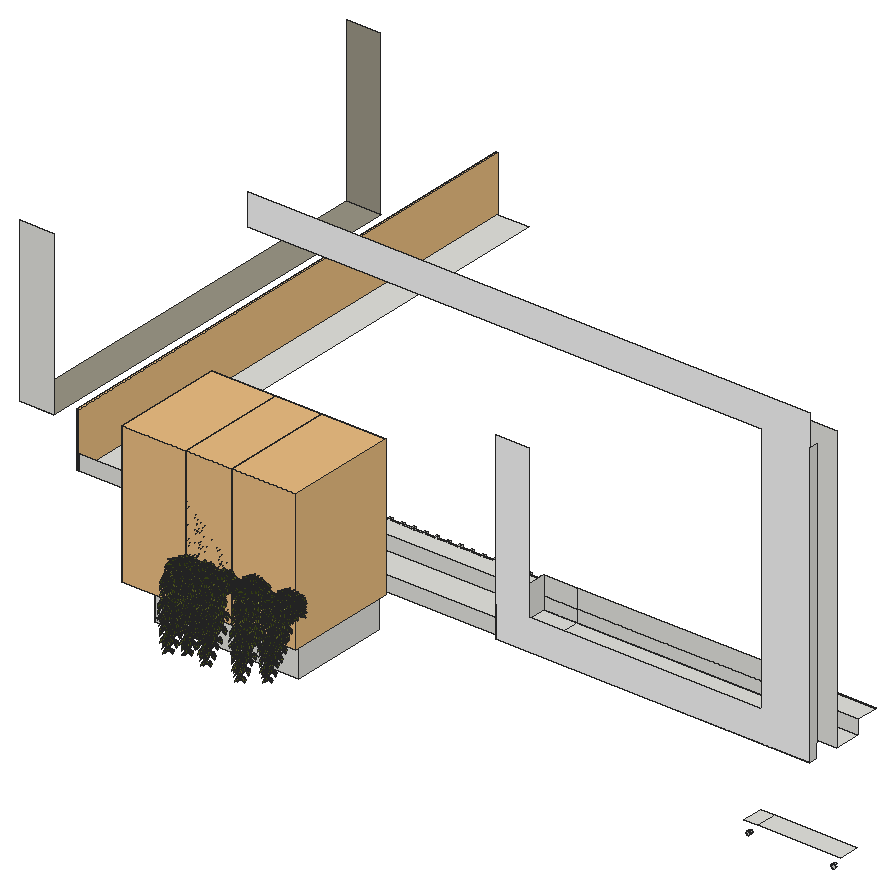
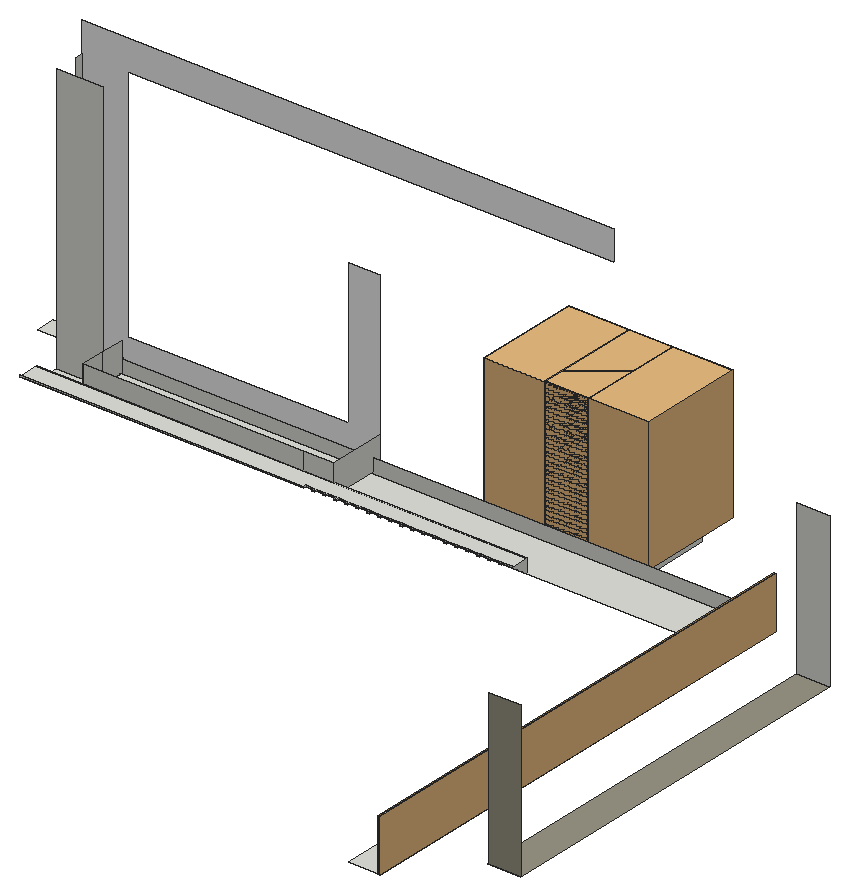
# SketchUp Ruby script. Lengths in inches.
U = 1.inch
M = Sketchup.active_model
def pt(a) = Geom::Point3d.new(a.map { |v| v * U })
def face(e, loops, mat)
  f = e.add_face(loops[0].map { |a| pt(a) })
  loops[1..].each { |l| e.add_face(l.map { |a| pt(a) }).erase! }
  f.material = f.back_material = mat if mat
  f
end
# faces: each face lists its corners as indices into pts; further lists are holes
def faces(e, pts, list, mat = nil) = list.each { |f| face(e, (f[0].is_a?(Array) ? f : [f]).map { |l| l.map { |i| pts[i] } }, mat) }
# xy, xz, yz: faces in a plane at the given z, y or x. An outline is a flat list of corners, or four numbers for a rectangle; further outlines are holes
def ring(l) = l.size == 4 ? [[l[0], l[1]], [l[2], l[1]], [l[2], l[3]], [l[0], l[3]]] : l.each_slice(2).to_a
def flat(e, list, mat, &to3) = list.each { |f| face(e, (f[0].is_a?(Array) ? f : [f]).map { |l| ring(l).map { |u, v| to3.(u, v) } }, mat) }
def xy(e, z, list, mat = nil) = flat(e, list, mat) { |x, y| [x, y, z] }
def xz(e, y, list, mat = nil) = flat(e, list, mat) { |x, z| [x, y, z] }
def yz(e, x, list, mat = nil) = flat(e, list, mat) { |y, z| [x, y, z] }
def lines(e, pts, list) = list.each { |a, b| e.add_line(pt(pts[a]), pt(pts[b])) }
# prism: a flat outline (further loops are holes) pulled along v
def prism(e, loops, v, mat = nil)
  f = face(e, loops, mat); d = Geom::Vector3d.new(v.map { |x| x * U })
  f.pushpull(f.normal.samedirection?(d) ? d.length : -d.length)
end
def box(e, o, s, mat = nil) = prism(e, [[o, [o[0] + s[0], o[1], o[2]], [o[0] + s[0], o[1] + s[1], o[2]], [o[0], o[1] + s[1], o[2]]]], [0, 0, s[2]], mat)
def at(x, y, z, deg = 0) = Geom::Transformation.translation(pt([x, y, z])) * Geom::Transformation.rotation(ORIGIN, Z_AXIS, deg.degrees)
def axes(o, x, y, z) = Geom::Transformation.new([*x, 0, *y, 0, *z, 0, *pt(o).to_a, 1])
def part(name) = M.definitions.add(name)
# library, detail: a bought-in or finely detailed component or shape, given as its bounding box
def library(name, o, s) = part(name).tap { |d| box(d.entities, o, s) }
def detail(e, o, s) = box(e.add_group.entities, o, s)
def put(e, d, t, mat = nil) = e.add_instance(d, t).tap { |i| i.material = mat if mat }
def group(e, t, mat = nil) = e.add_group.tap { |g| g.transformation = t; g.material = mat if mat }.entities
root = M.entities
M.materials.add("[0129_WhiteSmoke]1").color = [245, 245, 245]
M.materials.add("[Concrete Tile]").color = [155, 150, 134]
M.materials.add("asdfasdfasdfasdf").color = [186, 198, 91]
M.materials.add("leaf1_smaller_cleanasdfasfasdfas").color = [88, 95, 33]
M.materials.add("leaf2_smaller_cleansadfasdfasdfasd").color = [55, 66, 19]
c1 = part("glass-railing")
detail(c1.entities,[0,0,0],[1.26,75.59,33.1875])
c2 = library("plant (1)",[-35.72,-28.42,0],[66.31,67.39,84.38])
c3 = part("leaf1a")
p = [[1.06,3.74,11.78],[8.28,8.7,-0.64],[9.51,5.4,26.1],[17.76,4.04,11.26],[17.85,2.23,20],[14.31,3.29,26.73],
  [3.78,3.8125,25.98],[-0.21,2.38,19.72]]
faces(c3.entities,p,[[0,1,2],[2,1,3],[3,4,5],[3,5,2],[6,7,0],[0,2,6]],"leaf1_smaller_cleanasdfasfasdfas")
c4 = part("leaf2a")
p = [[1.4375,3.56,10.81],[8.71,6.8,-0.73],[9.51,3.5,26.59],[16.66,3.91,9.8],[17.86,1.3,19.21],[14.9,1.58,24.92],
  [5.15,2.55,24.01],[1.29,1.87,19.875]]
faces(c4.entities,p,[[0,1,2],[2,1,3],[3,4,5],[3,5,2],[6,7,0],[0,2,6]],"leaf2_smaller_cleansadfasdfasdfasd")
c5 = part("Group\#220")
put(c5.entities,c4,axes([6.68,1.92,2.42],[-0.04671,0.11082,0.08136],[0.07715,0.09226,-0.08136],[-0.11379,0.01705,-0.08856]))
put(c5.entities,c3,axes([1.26,0.54,1.25],[0.13756,-0.04533,0.01029],[0.0079,-0.00888,-0.14471],[0.04581,0.13766,-0.00594]))
put(c5.entities,c4,axes([-0.51,4.89,1.49],[-0.00057,-0.14139,-0.03304],[0.00922,0.03294,-0.14111],[0.14491,-0.00265,0.00885]))
put(c5.entities,c3,axes([4.37,7.98,1.26],[-0.14226,-0.02905,0],[0,0,-0.1452],[0.02905,-0.14226,0]))
put(c5.entities,c3,axes([1.46,4.03,4.07],[0.06242,-0.12847,-0.02614],[-0.10319,-0.03029,-0.09755],[0.08086,0.06051,-0.10432]))
c6 = part("leaf_a")
p = [[1.43,4.41,0.74],[1.39,4.36,0.69],[1.39,4.61,0.21],[1.43,4.67,0.24],[1.35,4.41,0.74],[1.35,4.67,0.24],
  [1.35,3.9,1.02],[1.43,3.9,1.02],[1.39,3.89,0.95],[1.39,3.35,0.9],[1.43,3.34,0.96],[1.35,3.34,0.96]]
faces(c6.entities,p,[[0,1,2,3],[1,4,5,2],[4,0,3,5],[3,2,5],[6,7,0,4],[8,6,4,1],[7,8,1,0],[9,10,11],
  [9,11,6,8],[10,9,8,7],[11,10,7,6]],"asdfasdfasdfasdf")
put(c6.entities,c4,axes([0,-0.08,0.875],[0.1452,0,0],[0,0.02746,-0.14258],[0,0.14258,0.02746]))
c7 = part("leaf_b")
prism(c7.entities,[[[1.36,4.21,-0.25],[1.31,4.13,-0.29],[1.26,4.21,-0.25]]],[0,-0.66,1.14],"asdfasdfasdfasdf")
put(c7.entities,c3,axes([0,-0.1,0.68],[0.1452,-0.0002,0],[0.00006,0.04124,-0.13922],[0.00019,0.13922,0.04124]))
c8 = part("Group\#209")
p = [[2.87,4.13,4.15],[2.98,3.98,4.12],[2.98,4.66,2.59],[2.87,4.8,2.65],[3.09,4.13,4.15],[3.09,4.8,2.65],
  [2.87,4.13,6.07],[2.98,3.98,6.12],[3.09,4.13,6.07],[2.87,5.04,7.34],[2.98,4.91,7.43],[3.09,5.04,7.34]]
faces(c8.entities,p,[[0,1,2,3],[1,4,5,2],[6,7,1,0],[7,8,4,1],[9,10,7,6],[10,11,8,7]],"asdfasdfasdfasdf")
put(c8.entities,c6,axes([0.86,0.51,1.53],[0.95176,-0.27809,0.12967],[0.18405,0.85554,0.48392],[-0.24551,-0.43671,0.86545]))
put(c8.entities,c7,axes([-0.97,2.96,6.52],[0.70711,-0.61237,-0.35355],[0.70711,0.61237,0.35355],[0,-0.5,0.86603]))
put(c8.entities,c6,axes([3.23,0.39,0.41],[0.82736,0.50176,-0.25242],[-0.32519,0.79434,0.5131],[0.45796,-0.34244,0.82037]))
put(c8.entities,c6,axes([3.25,-0.58,4.78],[0.8251,0.44069,-0.35355],[-0.31829,0.8796,0.35355],[0.46679,-0.17918,0.86603]))
c9 = part("Group\#2")
p = [[1.22,4.71,2.14],[1.31,4.57,2.14],[2.16,4.71,3.79],[2.24,4.57,3.77],[1.39,4.71,2.14],[2.33,4.71,3.79],
  [1.93,3.51,6.2],[1.85,3.64,6.23],[2.02,3.64,6.23],[0.93,3.38,8.58],[0.85,3.52,8.58],[1.02,3.52,8.58],
  [0.81,3.57,10.77],[0.72,3.71,10.73],[0.89,3.71,10.73],[1.31,4.57,13.2],[1.22,4.7,13.15],[1.39,4.7,13.15]]
faces(c9.entities,p,[[0,1,2],[3,2,1],[1,4,3],[5,3,4],[6,7,3],[6,3,8],[2,3,7],[5,8,3],
  [9,10,6],[9,6,11],[7,6,10],[8,11,6],[9,11,12],[9,12,10],[13,10,12],[14,12,11],
  [12,15,13],[12,14,15],[16,13,15],[17,15,14]],"asdfasdfasdfasdf")
put(c9.entities,c7,axes([3.93,1.17,1.97],[0.75139,0.49793,0.43299],[-0.65983,0.56085,0.50006],[0.00615,-0.66145,0.74997]))
put(c9.entities,c7,axes([6.23,5.09,1.92],[-0.36585,0.92196,0.12706],[-0.79398,-0.38042,0.47421],[0.48554,0.0726,0.87119]))
put(c9.entities,c7,axes([0.03,0.92,11.26],[1,0,0],[0,0.86603,0.5],[0,-0.5,0.86603]))
put(c9.entities,c6,axes([4.37,2.0625,9.11],[0.45529,0.76896,0.44879],[-0.86129,0.25267,0.44084],[0.22559,-0.58725,0.77733]))
put(c9.entities,c6,axes([1.89,-0.25,4.42],[0.88717,0.14116,0.43931],[-0.36372,0.79981,0.47751],[-0.28396,-0.58342,0.76091]))
put(c9.entities,c6,axes([-0.4,-0.0625,7.9],[0.80178,0.42258,-0.42258],[0,0.70711,0.70711],[0.59763,-0.56694,0.56694]))
put(c9.entities,c7,axes([0.05,0.6875,0.65],[0.97178,0.10445,-0.21151],[0.0126,0.87237,0.48869],[0.23556,-0.47756,0.84643]))
put(c9.entities,c6,axes([5.56,1.19,4.08],[0.24789,0.96746,-0.05068],[-0.86286,0.24427,0.4425],[0.44048,-0.06596,0.89533]))
put(c9.entities,c7,axes([4.91,2.14,7.29],[-0.04249,0.96546,-0.25705],[-0.89911,0.07524,0.4312],[0.43565,0.24944,0.86486]))
c10 = part("Group\#208")
put(c10.entities,c4,axes([5.59,5.52,3.3],[-0.07606,0.12201,-0.02028],[0.09645,0.0436,-0.0994],[-0.07744,-0.06554,-0.10388]))
put(c10.entities,c4,axes([7.69,4.27,1.08],[-0.09839,0.10661,0.00609],[-0.00698,0.00184,-0.14502],[-0.10656,-0.09856,0.00388]))
put(c10.entities,c3,axes([3.51,6.9,2.1],[-0.1403,-0.03711,-0.00465],[-0.00046,0.01976,-0.14385],[0.03739,-0.13898,-0.01921]))
put(c10.entities,c4,axes([2.18,0.07,1.375],[0.14025,0.00096,-0.03757],[-0.03758,0.00358,-0.14021],[0,0.14515,0.00371]))
put(c10.entities,c3,axes([-0.62,2,1.16],[0.081,-0.0806,-0.00996],[0.00004,0.01411,-0.11384],[0.08122,0.08039,0.00999]))
c11 = part("Group\#221")
p = [[1.22,4.71,2.14],[1.31,4.57,2.14],[2.16,4.71,3.79],[2.24,4.57,3.77],[1.39,4.71,2.14],[2.33,4.71,3.79],
  [1.93,3.51,6.2],[1.85,3.64,6.23],[2.02,3.64,6.23],[0.93,3.38,8.58],[0.85,3.52,8.58],[1.02,3.52,8.58],
  [0.81,3.57,10.77],[0.72,3.71,10.73],[0.89,3.71,10.73],[1.31,4.57,13.2],[1.22,4.7,13.15],[1.39,4.7,13.15]]
faces(c11.entities,p,[[0,1,2],[3,2,1],[1,4,3],[5,3,4],[6,7,3],[6,3,8],[2,3,7],[5,8,3],
  [9,10,6],[9,6,11],[7,6,10],[8,11,6],[9,11,12],[9,12,10],[13,10,12],[14,12,11],
  [12,15,13],[12,14,15],[16,13,15],[17,15,14]],"asdfasdfasdfasdf")
put(c11.entities,c7,axes([3.93,1.17,1.97],[0.75139,0.49793,0.43299],[-0.65983,0.56085,0.50006],[0.00615,-0.66145,0.74997]))
put(c11.entities,c7,axes([6.23,5.09,1.92],[-0.36585,0.92196,0.12706],[-0.79398,-0.38042,0.47421],[0.48554,0.0726,0.87119]))
put(c11.entities,c7,axes([0.03,0.92,11.26],[1,0,0],[0,0.86603,0.5],[0,-0.5,0.86603]))
put(c11.entities,c6,axes([4.37,2.0625,9.11],[0.45529,0.76896,0.44879],[-0.86129,0.25267,0.44084],[0.22559,-0.58725,0.77733]))
put(c11.entities,c6,axes([1.89,-0.25,4.42],[0.88717,0.14116,0.43931],[-0.36372,0.79981,0.47751],[-0.28396,-0.58342,0.76091]))
put(c11.entities,c6,axes([-0.4,-0.0625,7.9],[0.80178,0.42258,-0.42258],[0,0.70711,0.70711],[0.59763,-0.56694,0.56694]))
put(c11.entities,c7,axes([0.05,0.6875,0.65],[0.97178,0.10445,-0.21151],[0.0126,0.87237,0.48869],[0.23556,-0.47756,0.84643]))
put(c11.entities,c6,axes([5.56,1.19,4.08],[0.24789,0.96746,-0.05068],[-0.86286,0.24427,0.4425],[0.44048,-0.06596,0.89533]))
put(c11.entities,c7,axes([4.91,2.14,7.29],[-0.04249,0.96546,-0.25705],[-0.89911,0.07524,0.4312],[0.43565,0.24944,0.86486]))
c12 = part("Trailing philodendron")
put(c12.entities,c3,axes([3.65,12.52,19.68],[-0.0527,-0.13492,0.0101],[-0.03487,0.00307,-0.14092],[0.13073,-0.05357,-0.03351]))
put(c12.entities,c3,axes([5.13,11.34,20.6],[-0.03432,-0.12484,0.06572],[-0.08608,-0.03507,-0.11155],[0.11179,-0.06533,-0.06572]))
put(c12.entities,c4,axes([2.61,13.04,18.63],[0.05838,-0.12752,0.03758],[0.01564,-0.03417,-0.14025],[0.13202,0.06044,0]))
put(c12.entities,c4,axes([3.7,9.83,20.73],[-0.00129,-0.14519,0],[-0.0726,0.00064,-0.12575],[0.12574,-0.00112,-0.0726]))
put(c12.entities,c4,axes([11.375,11.11,20.23],[-0.14171,0.00126,0.03163],[-0.02867,0.05638,-0.1307],[-0.01341,-0.1338,-0.05478]))
put(c12.entities,c3,axes([2.4375,12.45,15.12],[-0.02375,-0.14324,0],[0.13106,-0.02173,-0.05859],[0.05781,-0.00958,0.13285]))
put(c12.entities,c3,axes([9.62,10.68,22.01],[0.05693,0.12487,-0.04742],[0.05061,-0.06787,-0.11796],[-0.12361,0.02972,-0.07014]))
put(c12.entities,c3,axes([11.63,16.35,20.5625],[-0.12691,-0.00762,0.07014],[-0.06947,0.03872,-0.12148],[-0.01233,-0.13973,-0.03749]))
put(c12.entities,c3,axes([12.51,17.52,17.81],[-0.1445,0.01001,0.0102],[-0.01383,-0.07182,-0.12544],[-0.0036,-0.1258,0.07242]))
put(c12.entities,c4,axes([9.09,6.34,22.72],[-0.09269,-0.05068,-0.09962],[-0.03661,0.13604,-0.03515],[0.1056,0.00268,-0.09962]))
put(c12.entities,c3,axes([4.83,12.62,22.54],[0.10783,0.09684,-0.00888],[0.09716,-0.10783,0.00397],[-0.00394,-0.00889,-0.14487]))
put(c12.entities,c3,axes([4.94,9.48,20.375],[0.01323,0.07633,0.07653],[0.10803,-0.00667,-0.01203],[-0.00375,0.07738,-0.07653]))
put(c12.entities,c4,axes([14,13.64,21.84],[-0.01852,-0.13907,0.03741],[-0.14373,0.01547,-0.01367],[0.00911,-0.03878,-0.13963]))
put(c12.entities,c4,axes([9.23,4.15,18.71],[0.14198,0.00177,-0.03038],[-0.02867,0.05638,-0.1307],[0.01021,0.13379,0.05548]))
put(c12.entities,c4,axes([5.82,4.5625,15.3],[0.13095,-0.05433,0.03137],[0.06268,0.11013,-0.07089],[0.00273,0.07747,0.12278]))
put(c12.entities,c5,axes([6.59,5.29,16.06],[1.23201,0.26412,0],[-0.26412,1.23201,0],[0,0,1.26]))
put(c12.entities,c8,axes([12.21,1.69,0.66],[-0.82914,0.03045,-0.02227],[0.02366,0.80139,0.21474],[-0.02938,-0.21389,0.80143]))
put(c12.entities,c9,axes([6.8125,1.15,7.57],[0.74375,-0.41052,0.02847],[0.41052,0.73612,-0.11],[0.02847,0.11,0.84237]))
put(c12.entities,c8,axes([-1.68,6.875,13.2],[0.5,-0.86603,0],[0.81585,0.47103,-0.33545],[0.29051,0.16773,0.94206]))
put(c12.entities,c8,axes([1.86,19.56,12.8125],[0.88164,0.4704,0.03781],[0.46333,-0.8476,-0.25863],[0.08962,-0.24554,0.96524]))
g1 = group(c12.entities,at(9.13,11.13,20.67))
put(g1,c4,axes([7.36,4.03,-0.3],[-0.05057,0.11966,-0.06487],[0.07036,-0.03625,-0.12173],[-0.11651,-0.07383,-0.04536]))
put(g1,c4,axes([8.4,1.56,-2.35],[-0.06703,0.12496,-0.03122],[-0.04831,-0.05702,-0.12449],[-0.1194,-0.04708,0.0679]))
put(g1,c3,axes([5.37,5.58,-2.1],[-0.14013,0.0124,0.03596],[-0.03803,-0.04347,-0.13322],[-0.00061,-0.13798,0.0452]))
put(g1,c4,axes([2.45,-0.07,0.8],[0.12002,-0.06072,-0.05468],[-0.07506,-0.04353,-0.11642],[0.03229,0.1245,-0.06737]))
put(g1,c3,axes([0.19,2.38,0.125],[0.05529,-0.09889,0.01797],[-0.03005,-0.03583,-0.10474],[0.09591,0.04578,-0.04318]))
put(c12.entities,c10,axes([17.33,10.54,16.15],[-0.62797,0.46654,0.62289],[-0.59637,-0.80271,0],[0.5,-0.37147,0.78231]))
put(c12.entities,c5,axes([3.44,11.88,17.73],[0.78616,-0.36326,0.5],[0.52263,0.82256,-0.22414],[-0.32986,0.43753,0.83652]))
put(c12.entities,c10,axes([5.5,5.07,16.54],[0.96593,-0.11102,0.2338],[0,0.90334,0.42894],[-0.25882,-0.41432,0.87255]))
put(c12.entities,c8,axes([18.84,3.62,12.91],[-0.80696,-0.59061,0],[-0.57048,0.77946,-0.25882],[-0.15286,0.20886,0.96593]))
put(c12.entities,c9,axes([3.89,0.96,5.21],[0.83948,0.00528,-0.02906],[-0.009,0.83292,-0.10846],[0.02813,0.1087,0.83246]))
put(c12.entities,c9,axes([6.1,0.84,-5.33],[0.875,-0.48296,0.03349],[0.48296,0.86603,-0.12941],[0.03349,0.12941,0.99103]))
put(c12.entities,c9,axes([3.87,-0.55,-8.84],[0.99938,0.00629,-0.0346],[-0.01071,0.99157,-0.12912],[0.03349,0.12941,0.99103]))
put(c12.entities,c8,axes([0.46,6.875,13.01],[0.5,-0.86603,0],[0.81585,0.47103,-0.33545],[0.29051,0.16773,0.94206]))
put(c12.entities,c9,axes([10.39,0.84,1.73],[0.875,-0.48296,0.03349],[0.48296,0.86603,-0.12941],[0.03349,0.12941,0.99103]))
put(c12.entities,c9,axes([-0.75,1.13,2.67],[0.7525,-0.41535,0.0288],[0.41535,0.74478,-0.11129],[0.0288,0.11129,0.85228]))
put(c12.entities,c9,axes([0.04,-0.97,-8.67],[0.735,-0.40569,0.02813],[0.40569,0.72746,-0.1087],[0.02813,0.1087,0.83246]))
put(c12.entities,c9,axes([0.09,-0.6,-7.42],[0.47403,-0.32078,-0.33698],[0.20171,0.57521,-0.26383],[0.41925,0.08595,0.50794]))
put(c12.entities,c9,axes([10.35,0.97,-6.0625],[0.76125,-0.42018,0.02914],[0.42018,0.75344,-0.11259],[0.02914,0.11259,0.86219]))
put(c12.entities,c9,axes([10.78,-1.55,-11.77],[0.72777,-0.42018,0.22517],[0.435,0.75344,0],[-0.19501,0.11259,0.84036]))
put(c12.entities,c9,axes([5.78,-1.55,-20.23],[0.76125,-0.42018,0.02914],[0.42018,0.75344,-0.11259],[0.02914,0.11259,0.86219]))
put(c12.entities,c9,axes([8.72,-1.43,-13.97],[0.65467,-0.36135,0.02506],[0.36135,0.64796,-0.09682],[0.02506,0.09682,0.74149]))
put(c12.entities,c11,axes([1.53,-0.97,-19.86],[0.735,-0.40569,0.02813],[0.40569,0.72746,-0.1087],[0.02813,0.1087,0.83246]))
put(c12.entities,c11,axes([6.23,-2.02,-7.18],[0.55125,-0.30427,0.0211],[0.39555,0.70927,-0.10599],[0.0211,0.08153,0.62435]))
put(c12.entities,c11,axes([6.43,-1.89,6.18],[0.735,-0.40569,0.02813],[0.5274,0.9457,-0.14132],[0.02813,0.1087,0.83246]))
put(c12.entities,c11,axes([10.24,1.09,9.64],[0.62475,-0.34484,0.02391],[0.44829,0.80384,-0.12012],[0.02391,0.0924,0.70759]))
put(c12.entities,c8,axes([1.56,7.74,12.8125],[-0.22619,0.97335,0.03781],[0.93864,0.22817,-0.25863],[0.26037,0.02301,0.96524]))
put(c12.entities,c8,axes([0.65,14.36,12.8125],[0.30411,0.95189,0.03781],[0.92309,-0.28464,-0.25863],[0.23543,-0.11355,0.96524]))
put(c12.entities,c8,axes([7.75,10.38,12.8125],[-0.84074,0.54011,0.03781],[0.51385,0.81797,-0.25863],[0.17062,0.19802,0.96524]))
put(c12.entities,c8,axes([12.92,19.16,12.8125],[0.9234,-0.38197,0.03781],[-0.36017,-0.89632,-0.25863],[-0.13268,-0.22521,0.96524]))
put(c12.entities,c8,axes([6.55,17.22,12.8125],[0.7985,0.60081,0.03781],[0.58857,-0.76596,-0.25863],[0.12643,-0.22877,0.96524]))
put(c12.entities,c8,axes([16.24,8.94,12.8125],[-0.64953,-0.75939,0.03781],[-0.7404,0.62041,-0.25863],[-0.17295,0.19599,0.96524]))
put(c12.entities,c8,axes([15.6875,15.74,12.8125],[0.12972,-0.99083,0.03781],[-0.95648,-0.13509,-0.25863],[-0.26137,0.00261,0.96524]))
put(c12.entities,c8,axes([19.85,8,15.61],[-0.64953,-0.75939,0.03781],[-0.7404,0.62041,-0.25863],[-0.17295,0.19599,0.96524]))
put(c12.entities,c8,axes([18.86,17.5,12.8125],[0.62831,-0.77705,0.03781],[-0.74495,-0.61494,-0.25863],[-0.22422,-0.13434,0.96524]))
put(c12.entities,c8,axes([-0.43,13.28,13.2],[-0.41945,-0.90778,0],[0.85518,-0.39515,-0.33545],[0.30452,-0.14071,0.94206]))
put(c12.entities,c11,axes([4.5625,-2.01,7.45],[0.56595,-0.31238,0.02166],[0.40609,0.72819,-0.10881],[0.02166,0.0837,0.641]))
put(c12.entities,c11,axes([4.48,-2.02,-24.24],[0.55125,-0.30427,0.0211],[0.39555,0.70927,-0.10599],[0.0211,0.08153,0.62435]))
put(c12.entities,c11,axes([4.9,-4.23,-11.04],[0.55125,-0.30427,0.0211],[0.39555,0.70927,-0.10599],[0.0211,0.08153,0.62435]))
put(c12.entities,c10,axes([17.33,10.54,17.41],[-0.62797,0.46654,0.62289],[-0.59637,-0.80271,0],[0.5,-0.37147,0.78231]))
put(c12.entities,c8,axes([-0.03,6.82,20.63],[0.44714,-0.87214,-0.19857],[0.53417,0.43844,-0.7228],[0.71744,0.21712,0.66191]))
put(c12.entities,c8,axes([20.82,12.8,12.8125],[0.12972,-0.99083,0.03781],[-0.95648,-0.13509,-0.25863],[-0.26137,0.00261,0.96524]))
xy(root,138.0625,[[848.72,801.78,857.125,814.22],[857.125,801.78,906.77,814.22]])
xy(root,138.1875,[[514,776.37,600.89,836.7]])
xy(root,153.5625,[[411.09,846.1,827.91,846.1,827.91,861.24,857.125,861.24,857.125,877.14,431.5,877.14,431.5,1160.85,411.09,1160.85]])
xy(root,154.75,[[667.84,840.97,687.49,877.14],[687.49,840.97,827.91,877.14],[827.91,840.97,857.125,845.35]])
xy(root,156.5,[[352.17,877.14,372.92,1122.97]],"[Concrete Tile]")
xy(root,162.125,[[545.16,877.14,545.16,888.95,550.57,888.95,550.57,890.39,552.22,890.39,552.22,888.95,557.63,888.95,557.63,890.39,559.22,890.39,559.22,888.95,564.63,888.95,564.63,890.39,566.22,890.39,566.22,888.95,571.63,888.95,571.63,890.39,573.22,890.39,573.22,888.95,578.63,888.95,578.63,890.39,580.22,890.39,580.22,888.95,585.63,888.95,585.63,890.39,587.22,890.39,587.22,888.95,592.63,888.95,592.63,890.39,594.22,890.39,594.22,888.95,599.63,888.95,599.63,890.39,601.22,890.39,601.22,888.95,606.63,888.95,606.63,890.39,608.22,890.39,608.22,888.95,613.63,888.95,613.63,890.39,615.22,890.39,615.22,888.95,620.63,888.95,620.63,890.39,622.22,890.39,622.22,888.95,627.63,888.95,627.63,890.39,629.22,890.39,629.22,888.95,634.63,888.95,634.63,890.39,636.22,890.39,636.22,888.83,641.63,888.83,641.63,890.39,643.22,890.39,643.22,888.83,648.63,888.83,648.63,890.39,650.22,890.39,650.22,888.83,655.63,888.83,655.63,890.39,657.22,890.39,657.22,888.83,662.63,888.83,662.63,890.39,664.22,890.39,664.22,888.83,669.63,888.83,669.63,890.39,671.22,890.39,671.22,888.83,676.63,888.83,676.63,890.39,857.125,890.39,857.125,877.14]])
xz(root,776.37,[[514,138.1875,600.89,183.3125]])
xz(root,799.91,[[852.61,131.88,852.9,131.92,853.17,132.03,853.4,132.21,853.58,132.44,853.69,132.71,853.73,133,853.69,133.29,853.58,133.57,853.4,133.8,853.17,133.98,852.9,134.09,852.61,134.13,852.32,134.09,852.05,133.98,851.8125,133.8,851.63,133.57,851.52,133.29,851.48,133,851.52,132.71,851.63,132.44,851.8125,132.21,852.05,132.03,852.32,131.92],[903.73,131.88,904.02,131.92,904.3,132.03,904.53,132.21,904.71,132.44,904.82,132.71,904.86,133,904.82,133.29,904.71,133.57,904.53,133.8,904.3,133.98,904.02,134.09,903.73,134.13,903.44,134.09,903.17,133.98,902.9375,133.8,902.76,133.57,902.65,133.29,902.61,133,902.65,132.71,902.76,132.44,902.9375,132.21,903.17,132.03,903.44,131.92]])
xz(root,836.7,[[514,138.1875,600.89,183.3125]])
xz(root,840.97,[[667.84,154.75,857.125,154.75,857.125,343.4375,518.47,343.4375,518.47,324.5625,827.91,324.5625,827.91,173.4375,687.49,173.4375,687.49,264.75,667.84,264.75]],"[0129_WhiteSmoke]1")
xz(root,845.35,[[827.91,154.75,857.125,163]])
xz(root,846.1,[[411.09,153.5625,827.91,162.75]])
xz(root,861.24,[[827.91,153.5625,857.125,324.5625]])
xz(root,877.14,[[545.16,153.5625,857.125,153.5625,857.125,162.125,827.91,162.125,827.91,154.75,667.84,154.75,667.84,162.125,545.16,162.125],[667.84,154.75,687.49,162.125],[687.49,154.75,827.91,162.125],[352.17,156.5,372.92,254.125],[667.84,162.125,687.49,173.4375],
  [687.49,162.125,827.91,173.4375]])
xz(root,888.83,[[636.22,162.125,641.63,162.75],[643.22,162.125,648.63,162.75],[650.22,162.125,655.63,162.75],[657.22,162.125,662.63,162.75],[664.22,162.125,669.63,162.75],
  [671.22,162.125,676.63,162.75]])
xz(root,888.95,[[545.16,162.125,550.57,162.75],[552.22,162.125,557.63,162.75],[559.22,162.125,564.63,162.75],[566.22,162.125,571.63,162.75],[573.22,162.125,578.63,162.75],
  [580.22,162.125,585.63,162.75],[587.22,162.125,592.63,162.75],[594.22,162.125,599.63,162.75],[601.22,162.125,606.63,162.75],[608.22,162.125,613.63,162.75],
  [615.22,162.125,620.63,162.75],[622.22,162.125,627.63,162.75],[629.22,162.125,634.63,162.75]])
xz(root,890.39,[[550.57,162.125,552.22,162.75],[557.63,162.125,559.22,162.75],[564.63,162.125,566.22,162.75],[571.63,162.125,573.22,162.75],[578.63,162.125,580.22,162.75],
  [585.63,162.125,587.22,162.75],[592.63,162.125,594.22,162.75],[599.63,162.125,601.22,162.75],[606.63,162.125,608.22,162.75],[613.63,162.125,615.22,162.75],
  [620.63,162.125,622.22,162.75],[627.63,162.125,629.22,162.75],[634.63,162.125,636.22,162.75],[641.63,162.125,643.22,162.75],[648.63,162.125,650.22,162.75],
  [655.63,162.125,657.22,162.75],[662.63,162.125,664.22,162.75],[669.63,162.125,671.22,162.75],[676.63,162.125,679.76,162.75],[679.76,162.125,857.125,162.75]])
xz(root,1122.97,[[352.17,156.5,372.3,254.125]],"[Concrete Tile]")
yz(root,514,[[776.37,138.1875,836.7,183.3125]])
yz(root,550.57,[[888.95,162.125,890.39,162.75]])
yz(root,552.22,[[888.95,162.125,890.39,162.75]])
yz(root,557.63,[[888.95,162.125,890.39,162.75]])
yz(root,559.22,[[888.95,162.125,890.39,162.75]])
yz(root,564.63,[[888.95,162.125,890.39,162.75]])
yz(root,566.22,[[888.95,162.125,890.39,162.75]])
yz(root,571.63,[[888.95,162.125,890.39,162.75]])
yz(root,573.22,[[888.95,162.125,890.39,162.75]])
yz(root,578.63,[[888.95,162.125,890.39,162.75]])
yz(root,580.22,[[888.95,162.125,890.39,162.75]])
yz(root,585.63,[[888.95,162.125,890.39,162.75]])
yz(root,587.22,[[888.95,162.125,890.39,162.75]])
yz(root,592.63,[[888.95,162.125,890.39,162.75]])
yz(root,594.22,[[888.95,162.125,890.39,162.75]])
yz(root,599.63,[[888.95,162.125,890.39,162.75]])
yz(root,600.89,[[776.37,138.1875,836.7,183.3125]])
yz(root,601.22,[[888.95,162.125,890.39,162.75]])
yz(root,606.63,[[888.95,162.125,890.39,162.75]])
yz(root,608.22,[[888.95,162.125,890.39,162.75]])
yz(root,613.63,[[888.95,162.125,890.39,162.75]])
yz(root,615.22,[[888.95,162.125,890.39,162.75]])
yz(root,620.63,[[888.95,162.125,890.39,162.75]])
yz(root,622.22,[[888.95,162.125,890.39,162.75]])
yz(root,627.63,[[888.95,162.125,890.39,162.75]])
yz(root,629.22,[[888.95,162.125,890.39,162.75]])
yz(root,634.63,[[888.95,162.125,890.39,162.75]])
yz(root,636.22,[[888.83,162.125,890.39,162.75]])
yz(root,641.63,[[888.83,162.125,890.39,162.75]])
yz(root,643.22,[[888.83,162.125,890.39,162.75]])
yz(root,648.63,[[888.83,162.125,890.39,162.75]])
yz(root,650.22,[[888.83,162.125,890.39,162.75]])
yz(root,655.63,[[888.83,162.125,890.39,162.75]])
yz(root,657.22,[[888.83,162.125,890.39,162.75]])
yz(root,662.63,[[888.83,162.125,890.39,162.75]])
yz(root,664.22,[[888.83,162.125,890.39,162.75]])
yz(root,667.84,[[840.97,154.75,877.14,173.4375]])
yz(root,669.63,[[888.83,162.125,890.39,162.75]])
yz(root,671.22,[[888.83,162.125,890.39,162.75]])
yz(root,676.63,[[888.83,162.125,890.39,162.75]])
yz(root,827.91,[[846.1,153.5625,861.24,154.75],[845.35,154.75,846.1,162.75],[846.1,154.75,861.24,173.4375],[861.24,154.75,877.14,173.4375]])
yz(root,857.125,[[840.97,154.75,845.35,154.75,845.35,163,846.1,163,846.1,324.5625,840.97,324.5625]])
p = [[852.05,801.78,132.03],[852.32,801.78,131.92],[852.32,799.91,131.92],[852.05,799.91,132.03],[852.61,801.78,131.88],[852.61,799.91,131.88],
  [852.9,801.78,131.92],[852.9,799.91,131.92],[853.17,801.78,132.03],[853.17,799.91,132.03],[903.17,801.78,132.03],[903.44,801.78,131.92],
  [903.44,799.91,131.92],[903.17,799.91,132.03],[903.73,801.78,131.88],[903.73,799.91,131.88],[904.02,801.78,131.92],[904.02,799.91,131.92],
  [904.3,801.78,132.03],[904.3,799.91,132.03],[851.8125,801.78,132.21],[851.8125,799.91,132.21],[853.4,801.78,132.21],[853.4,799.91,132.21],
  [902.9375,801.78,132.21],[902.9375,799.91,132.21],[904.53,801.78,132.21],[904.53,799.91,132.21],[851.63,801.78,132.44],[851.63,799.91,132.44],
  [853.58,801.78,132.44],[853.58,799.91,132.44],[902.76,801.78,132.44],[902.76,799.91,132.44],[851.52,801.78,132.71],[851.52,799.91,132.71],
  [853.69,801.78,132.71],[853.69,799.91,132.71],[902.65,801.78,132.71],[902.65,799.91,132.71],[851.48,801.78,133],[851.48,799.91,133],
  [853.73,801.78,133],[853.73,799.91,133],[902.61,801.78,133],[902.61,799.91,133],[851.52,801.78,133.29],[851.52,799.91,133.29],
  [853.69,801.78,133.29],[853.69,799.91,133.29],[902.65,801.78,133.29],[902.65,799.91,133.29],[851.63,801.78,133.57],[851.63,799.91,133.57],
  [853.58,801.78,133.57],[853.58,799.91,133.57],[902.76,801.78,133.57],[902.76,799.91,133.57],[851.8125,801.78,133.8],[851.8125,799.91,133.8],
  [853.4,801.78,133.8],[853.4,799.91,133.8],[902.9375,801.78,133.8],[902.9375,799.91,133.8],[852.05,801.78,133.98],[852.05,799.91,133.98],
  [853.17,801.78,133.98],[853.17,799.91,133.98],[903.17,801.78,133.98],[903.17,799.91,133.98],[852.32,801.78,134.09],[852.32,799.91,134.09],
  [852.9,801.78,134.09],[852.9,799.91,134.09],[903.44,801.78,134.09],[903.44,799.91,134.09],[904.3,801.78,133.98],[904.02,801.78,134.09],
  [904.02,799.91,134.09],[904.3,799.91,133.98],[852.61,801.78,134.13],[852.61,799.91,134.13],[903.73,801.78,134.13],[903.73,799.91,134.13]]
faces(root,p,[[0,1,2,3],[1,4,5,2],[4,6,7,5],[6,8,9,7],[10,11,12,13],[11,14,15,12],[14,16,17,15],[16,18,19,17],
  [20,0,3,21],[8,22,23,9],[24,10,13,25],[18,26,27,19],[28,20,21,29],[22,30,31,23],[32,24,25,33],[34,28,29,35],
  [30,36,37,31],[38,32,33,39],[40,34,35,41],[36,42,43,37],[44,38,39,45],[46,40,41,47],[42,48,49,43],[50,44,45,51],
  [52,46,47,53],[48,54,55,49],[56,50,51,57],[58,52,53,59],[54,60,61,55],[62,56,57,63],[64,58,59,65],[60,66,67,61],
  [68,62,63,69],[70,64,65,71],[66,72,73,67],[74,68,69,75],[76,77,78,79],[80,70,71,81],[72,80,81,73],[82,74,75,83],
  [77,82,83,78]])
put(root,c1,axes([411.09,846.1,153.5625],[1,0,0],[0,4.1738,0],[0,0,1]))
put(root,c2,at(533.01,800.97,155.86))
put(root,c12,axes([530.13,757.41,163.27],[1.02772,-0.11891,0],[0.11891,1.02772,0],[0,0,1.03457]))
put(root,c12,axes([541.35,758.42,164.63],[0.97878,-0.11325,0],[0.11325,0.97878,0],[0,0,0.98531]))
put(root,c12,axes([552.68,757.84,163.85],[1.00674,-0.11648,0],[0.11648,1.00674,0],[0,0,1.01346]))
put(root,c2,at(571.58,800.97,155.86))
put(root,c12,axes([571.8,764.1875,172.43],[0.69913,-0.08089,0],[0.08089,0.69913,0],[0,0,0.70379]))
put(root,c12,axes([573.38,757.41,163.27],[1.02772,-0.11891,0],[0.11891,1.02772,0],[0,0,1.03457]))
put(root,c12,axes([588.35,760.14,164.61],[0.94382,-0.1092,0],[0.1092,0.94382,0],[0,0,0.95012]))
put(root,c12,axes([593.05,764.1875,172.43],[0.69913,-0.08089,0],[0.08089,0.69913,0],[0,0,0.70379]))
